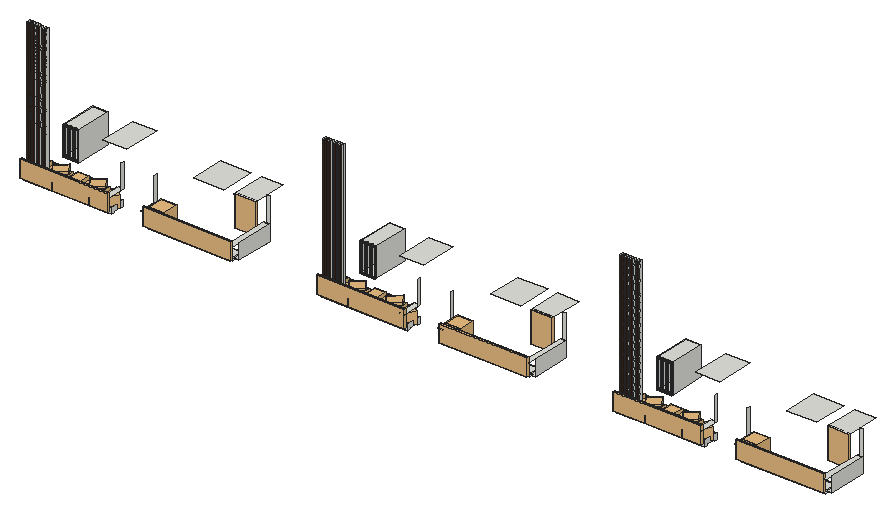
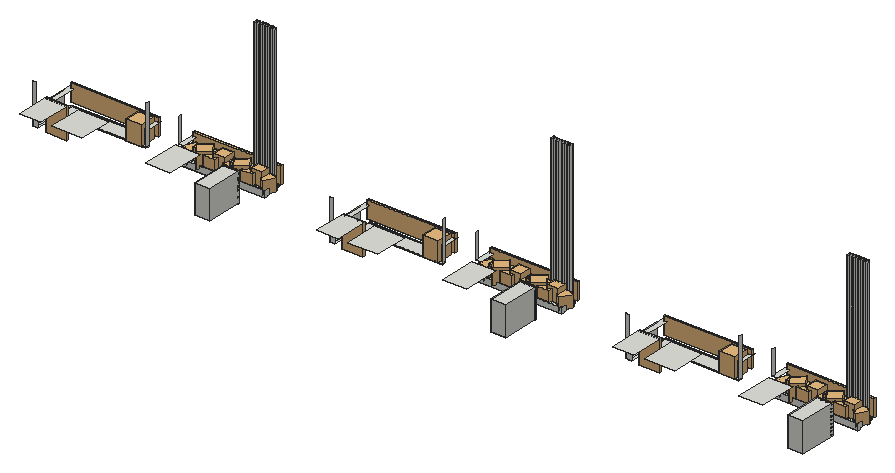
# SketchUp Ruby script. Lengths in inches.
U = 1.inch
M = Sketchup.active_model
def pt(a) = Geom::Point3d.new(a.map { |v| v * U })
def face(e, loops, mat)
  f = e.add_face(loops[0].map { |a| pt(a) })
  loops[1..].each { |l| e.add_face(l.map { |a| pt(a) }).erase! }
  f.material = f.back_material = mat if mat
  f
end
# faces: each face lists its corners as indices into pts; further lists are holes
def faces(e, pts, list, mat = nil) = list.each { |f| face(e, (f[0].is_a?(Array) ? f : [f]).map { |l| l.map { |i| pts[i] } }, mat) }
# xy, xz, yz: faces in a plane at the given z, y or x. An outline is a flat list of corners, or four numbers for a rectangle; further outlines are holes
def ring(l) = l.size == 4 ? [[l[0], l[1]], [l[2], l[1]], [l[2], l[3]], [l[0], l[3]]] : l.each_slice(2).to_a
def flat(e, list, mat, &to3) = list.each { |f| face(e, (f[0].is_a?(Array) ? f : [f]).map { |l| ring(l).map { |u, v| to3.(u, v) } }, mat) }
def xy(e, z, list, mat = nil) = flat(e, list, mat) { |x, y| [x, y, z] }
def xz(e, y, list, mat = nil) = flat(e, list, mat) { |x, z| [x, y, z] }
def yz(e, x, list, mat = nil) = flat(e, list, mat) { |y, z| [x, y, z] }
def lines(e, pts, list) = list.each { |a, b| e.add_line(pt(pts[a]), pt(pts[b])) }
# prism: a flat outline (further loops are holes) pulled along v
def prism(e, loops, v, mat = nil)
  f = face(e, loops, mat); d = Geom::Vector3d.new(v.map { |x| x * U })
  f.pushpull(f.normal.samedirection?(d) ? d.length : -d.length)
end
def box(e, o, s, mat = nil) = prism(e, [[o, [o[0] + s[0], o[1], o[2]], [o[0] + s[0], o[1] + s[1], o[2]], [o[0], o[1] + s[1], o[2]]]], [0, 0, s[2]], mat)
def at(x, y, z, deg = 0) = Geom::Transformation.translation(pt([x, y, z])) * Geom::Transformation.rotation(ORIGIN, Z_AXIS, deg.degrees)
def axes(o, x, y, z) = Geom::Transformation.new([*x, 0, *y, 0, *z, 0, *pt(o).to_a, 1])
def part(name) = M.definitions.add(name)
# library, detail: a bought-in or finely detailed component or shape, given as its bounding box
def library(name, o, s) = part(name).tap { |d| box(d.entities, o, s) }
def detail(e, o, s) = box(e.add_group.entities, o, s)
def put(e, d, t, mat = nil) = e.add_instance(d, t).tap { |i| i.material = mat if mat }
def group(e, t, mat = nil) = e.add_group.tap { |g| g.transformation = t; g.material = mat if mat }.entities
root = M.entities
M.materials.add("Material__1").color = [95, 70, 46]
M.materials.add("Wine2").color = [0, 0, 0]
M.materials["Wine2"].alpha = 0
M.materials.add("[0130_Gainsboro]").color = [39, 45, 50]
M.materials.add("[Wood Floor Parquet]").color = [140, 85, 37]
M.materials.add("[Wood Veneer 01]").color = [51, 28, 15]
c1 = library("Areca palm plant",[0,0,0],[49.1,36.6,54.46])
c2 = library("Group\#74",[-84.69,-90.07,-0.36],[176.51,175.13,171.4])
c3 = library("Group20\#1",[-20.81,-17.08,3.79],[39.86,39.43,37.51])
c4 = library("Group\#130",[-7.34,-1.2,0],[38.67,35.81,49.04])
c5 = library("Group38\#2",[14.01,28.44,-23.43],[18.58,18.32,38.89])
c6 = part("Group\#16")
put(c6.entities,c1,axes([-6.2,158.41,6.08],[0.45017,-0.56191,0],[0.66137,0.52986,0],[0,0,0.72]))
put(c6.entities,c1,axes([-6.2,56.6,6.08],[0.45017,-0.56191,0],[0.66137,0.52986,0],[0,0,0.72]))
put(c6.entities,c2,axes([14.93,145.87,6.05],[-0.04961,-0.08593,0],[0.08593,-0.04961,0],[0,0,0.10522]))
put(c6.entities,c3,axes([18.97,79.98,4.77],[0,0.85,0],[-0.85,0,0],[0,0,0.85]))
put(c6.entities,c2,axes([14.93,173.12,6.05],[-0.04961,-0.08593,0],[0.08593,-0.04961,0],[0,0,0.10522]))
put(c6.entities,c2,axes([14.93,193.18,6.05],[-0.04961,-0.08593,0],[0.08593,-0.04961,0],[0,0,0.10522]))
put(c6.entities,c4,axes([24.9375,89.91,8],[0,0.79,0],[-0.79,0,0],[0,0,0.79]))
put(c6.entities,c5,axes([-4.1,-1.15,28.17],[0.8848,0,0],[0,0.94674,0],[0,0,0.85826]))
g1 = group(c6.entities,at(0,0,0))
xy(g1,0,[[0,0,6,234.8],[30,0,36,234.8]])
xy(g1,3,[[6,0,30,234.8]])
xy(g1,7,[[6,5,30,229.8]],"Material__1")
xy(g1,15,[[[0,0,36,234.8],[6,5,30,229.8]]])
xz(g1,0,[[0,0,6,0,6,3,30,3,30,0,36,0,36,15,0,15]])
xz(g1,5,[[6,7,30,15]])
xz(g1,229.8,[[6,7,30,15]])
xz(g1,234.8,[[0,0,0,15,36,15,36,0,30,0,30,3,6,3,6,0]])
yz(g1,0,[[0,0,234.8,15]])
yz(g1,6,[[0,0,234.8,3],[5,7,229.8,15]])
yz(g1,30,[[0,0,234.8,3],[5,7,229.8,15]])
yz(g1,36,[[0,0,234.8,15]])
put(c6.entities,c2,axes([14.93,91.37,6.05],[-0.04961,-0.08593,0],[0.08593,-0.04961,0],[0,0,0.10522]))
put(c6.entities,c2,axes([14.93,44.05,6.05],[-0.04961,-0.08593,0],[0.08593,-0.04961,0],[0,0,0.10522]))
put(c6.entities,c4,axes([24.9375,191.72,8],[0,0.79,0],[-0.79,0,0],[0,0,0.79]))
put(c6.entities,c5,axes([-4.1,100.66,28.17],[0.8848,0,0],[0,0.94674,0],[0,0,0.85826]))
put(c6.entities,c2,axes([17.19,15.79,6.07],[-0.08133,-0.14087,0],[0.14087,-0.08133,0],[0,0,0.1725]))
put(c6.entities,c2,axes([14.93,71.3,6.05],[-0.04961,-0.08593,0],[0.08593,-0.04961,0],[0,0,0.10522]))
put(c6.entities,c2,axes([17.19,121.23,6.07],[-0.08133,-0.14087,0],[0.14087,-0.08133,0],[0,0,0.1725]))
put(c6.entities,c2,axes([17.19,223.04,6.07],[-0.08133,-0.14087,0],[0.14087,-0.08133,0],[0,0,0.1725]))
put(c6.entities,c3,axes([18.97,181.79,4.77],[0,0.85,0],[-0.85,0,0],[0,0,0.85]))
c7 = library("元件\#5",[-4.39,0,0],[5.37,35.83,90.55])
c8 = library("plant (1)",[-35.72,-28.42,0],[66.31,67.39,84.38])
c9 = library("Glass Railing",[0,0,0],[139.5,4.76,42])
c10 = part("Group\#55")
xy(c10.entities,0,[[0,-0.98,43.07,0],[0,0,43.07,1.4]],"[0130_Gainsboro]")
xy(c10.entities,0.3,[[0.3,-1.43,42.77,-0.98]],"[0130_Gainsboro]")
xy(c10.entities,2.95,[[2.95,-1.43,40.12,-0.63],[2.95,-0.63,40.12,0],[2.95,0,40.12,0.64],[2.95,0.64,40.12,1.4]],"[0130_Gainsboro]")
xy(c10.entities,3.54,[[3.54,-0.63,39.53,0],[3.54,0,39.53,0.64]],"[0130_Gainsboro]")
xy(c10.entities,111.8125,[[3.54,-0.63,39.53,0],[3.54,0,39.53,0.64]],"[0130_Gainsboro]")
xy(c10.entities,112.4,[[2.95,-1.43,40.12,-0.63],[2.95,-0.63,40.12,0],[2.95,0,40.12,0.64],[2.95,0.64,40.12,1.4]],"[0130_Gainsboro]")
xy(c10.entities,115.05,[[0.3,-1.43,42.77,-0.98]],"[0130_Gainsboro]")
xy(c10.entities,115.35,[[0,-0.98,43.07,0],[0,0,43.07,1.4]],"[0130_Gainsboro]")
xz(c10.entities,-1.43,[[[0.3,0.3,42.77,115.05],[2.95,2.95,40.12,112.4]]],"[Wood Veneer 01]")
xz(c10.entities,-0.98,[[[0,0,43.07,115.35],[0.3,0.3,42.77,115.05]]],"[0130_Gainsboro]")
xz(c10.entities,-0.63,[[[2.95,2.95,40.12,112.4],[3.54,3.54,39.53,111.8125]]],"[0130_Gainsboro]")
xz(c10.entities,0,[[3.54,3.54,39.53,111.8125]],"Wine2")
xz(c10.entities,0,[[[0,0,43.07,115.35],[2.95,2.95,40.12,112.4]],[[2.95,2.95,40.12,112.4],[3.54,3.54,39.53,111.8125]]],"[0130_Gainsboro]")
xz(c10.entities,0.64,[[[2.95,2.95,40.12,112.4],[3.54,3.54,39.53,111.8125]]],"[0130_Gainsboro]")
xz(c10.entities,1.4,[[[0,0,43.07,115.35],[2.95,2.95,40.12,112.4]]],"[0130_Gainsboro]")
yz(c10.entities,0,[[-0.98,0,0,115.35],[0,0,1.4,115.35]],"[0130_Gainsboro]")
yz(c10.entities,0.3,[[-1.43,0.3,-0.98,115.05]],"[0130_Gainsboro]")
yz(c10.entities,2.95,[[-1.43,2.95,-0.63,112.4],[-0.63,2.95,0,112.4],[0,2.95,0.64,112.4],[0.64,2.95,1.4,112.4]],"[0130_Gainsboro]")
yz(c10.entities,3.54,[[-0.63,3.54,0,111.8125],[0,3.54,0.64,111.8125]],"[0130_Gainsboro]")
yz(c10.entities,39.53,[[-0.63,3.54,0,111.8125],[0,3.54,0.64,111.8125]],"[0130_Gainsboro]")
yz(c10.entities,40.12,[[-1.43,2.95,-0.63,112.4],[-0.63,2.95,0,112.4],[0,2.95,0.64,112.4],[0.64,2.95,1.4,112.4]],"[0130_Gainsboro]")
yz(c10.entities,42.77,[[-1.43,0.3,-0.98,115.05]],"[0130_Gainsboro]")
yz(c10.entities,43.07,[[-0.98,0,0,115.35],[0,0,1.4,115.35]],"[0130_Gainsboro]")
c11 = part("Component\#21")
put(c11.entities,c10,axes([90.57,1.43,0],[1.05148,0,0],[0,1,0],[0,0,1]))
put(c11.entities,c10,axes([0,1.43,0],[1.05148,0,0],[0,1,0],[0,0,1]))
put(c11.entities,c10,axes([45.29,1.43,0],[1.05148,0,0],[0,1,0],[0,0,1]),"[Wood Veneer 01]")
xy(root,154.75,[[100.18,254.22,106.73,256.84],[106.73,254.22,113.67,256.84],[113.67,254.22,119.31,256.84],[119.31,254.22,126.24,256.84],[126.24,254.22,132.68,256.84],
  [132.68,254.22,139.62,256.84],[139.62,254.22,146.56,256.84],[146.56,254.22,153.49,256.84],[153.49,254.22,303.41,256.84],[409.32,254.22,409.32,255.72,412.47,255.72,412.47,256.84,609.07,256.84,609.07,254.22],
  [833.74,254.22,840.29,256.84],[840.29,254.22,847.23,256.84],[847.23,254.22,852.87,256.84],[852.87,254.22,859.81,256.84],[859.81,254.22,866.24,256.84],
  [866.24,254.22,873.18,256.84],[873.18,254.22,880.12,256.84],[880.12,254.22,887.06,256.84],[887.06,254.22,1036.98,256.84],[1142.89,254.22,1142.89,255.72,1146.03,255.72,1146.03,256.84,1342.64,256.84,1342.64,254.22],
  [1567.3,254.22,1573.86,256.84],[1573.86,254.22,1580.79,256.84],[1580.79,254.22,1586.43,256.84],[1586.43,254.22,1593.37,256.84],[1593.37,254.22,1599.81,256.84],
  [1599.81,254.22,1606.74,256.84],[1606.74,254.22,1613.68,256.84],[1613.68,254.22,1620.62,256.84],[1620.62,254.22,1770.54,256.84],[1876.45,254.22,1876.45,255.72,1879.6,255.72,1879.6,256.84,2076.2,256.84,2076.2,254.22],
  [100.18,256.84,100.18,275.15,303.41,275.15,303.41,256.84,153.49,256.84,153.49,263.78,146.56,263.78,146.56,256.84,139.62,256.84,139.62,263.78,132.68,263.78,132.68,256.84,126.24,256.84,126.24,263.78,119.31,263.78,119.31,256.84,113.67,256.84,113.67,263.78,106.73,263.78,106.73,256.84],[106.73,256.84,113.67,263.78],[119.31,256.84,126.24,263.78],[132.68,256.84,139.62,263.78],[146.56,256.84,153.49,263.78],
  [409.32,256.84,409.32,286.21,396.57,286.21,396.57,293.45,609.07,293.45,609.07,256.84],[609.07,256.84,614.76,266.43],[833.74,256.84,833.74,275.15,1036.98,275.15,1036.98,256.84,887.06,256.84,887.06,263.78,880.12,263.78,880.12,256.84,873.18,256.84,873.18,263.78,866.24,263.78,866.24,256.84,859.81,256.84,859.81,263.78,852.87,263.78,852.87,256.84,847.23,256.84,847.23,263.78,840.29,263.78,840.29,256.84],[840.29,256.84,847.23,263.78],[852.87,256.84,859.81,263.78],
  [866.24,256.84,873.18,263.78],[880.12,256.84,887.06,263.78],[1142.89,256.84,1142.89,286.21,1130.14,286.21,1130.14,293.45,1342.64,293.45,1342.64,256.84],[1342.64,256.84,1348.32,266.43],[1567.3,256.84,1567.3,275.15,1770.54,275.15,1770.54,256.84,1620.62,256.84,1620.62,263.78,1613.68,263.78,1613.68,256.84,1606.74,256.84,1606.74,263.78,1599.81,263.78,1599.81,256.84,1593.37,256.84,1593.37,263.78,1586.43,263.78,1586.43,256.84,1580.79,256.84,1580.79,263.78,1573.86,263.78,1573.86,256.84],
  [1573.86,256.84,1580.79,263.78],[1586.43,256.84,1593.37,263.78],[1599.81,256.84,1606.74,263.78],[1613.68,256.84,1620.62,263.78],[1876.45,256.84,1876.45,286.21,1863.7,286.21,1863.7,293.45,2076.2,293.45,2076.2,256.84],
  [2076.2,256.84,2081.89,266.43],[609.07,266.43,609.07,293.45,614.76,293.45,614.76,361.27,622,361.27,622,266.43],[1342.64,266.43,1342.64,293.45,1348.32,293.45,1348.32,361.27,1355.5625,361.27,1355.5625,266.43],[2076.2,266.43,2076.2,293.45,2081.89,293.45,2081.89,361.27,2089.125,361.27,2089.125,266.43],[609.07,293.45,614.76,361.27],
  [1342.64,293.45,1348.32,361.27],[2076.2,293.45,2081.89,361.27]])
xy(root,154.75,[[409.32,255.72,412.47,256.78],[1142.89,255.72,1146.03,256.78],[1876.45,255.72,1879.6,256.78],[409.32,256.78,412.47,256.84],[1142.89,256.78,1146.03,256.84],
  [1876.45,256.78,1879.6,256.84]],"[Wood Veneer 01]")
xy(root,156.9375,[[409.32,254.22,609.07,256.84],[1142.89,254.22,1342.64,256.84],[1876.45,254.22,2076.2,256.84],[409.32,256.84,609.07,256.84,609.07,293.45,396.57,293.45,396.57,286.21,409.32,286.21],[1142.89,256.84,1342.64,256.84,1342.64,293.45,1130.14,293.45,1130.14,286.21,1142.89,286.21],
  [1876.45,256.84,2076.2,256.84,2076.2,293.45,1863.7,293.45,1863.7,286.21,1876.45,286.21]])
xy(root,158.1875,[[100.18,254.22,106.73,256.84],[113.67,254.22,119.31,256.84],[126.24,254.22,132.68,256.84],[139.62,254.22,146.56,256.84],[153.49,254.22,303.41,256.84],
  [833.74,254.22,840.29,256.84],[847.23,254.22,852.87,256.84],[859.81,254.22,866.24,256.84],[873.18,254.22,880.12,256.84],[887.06,254.22,1036.98,256.84],
  [1567.3,254.22,1573.86,256.84],[1580.79,254.22,1586.43,256.84],[1593.37,254.22,1599.81,256.84],[1606.74,254.22,1613.68,256.84],[1620.62,254.22,1770.54,256.84],
  [100.18,256.84,106.73,256.84,106.73,263.78,113.67,263.78,113.67,256.84,119.31,256.84,119.31,263.78,126.24,263.78,126.24,256.84,132.68,256.84,132.68,263.78,139.62,263.78,139.62,256.84,146.56,256.84,146.56,263.78,153.49,263.78,153.49,256.84,303.41,256.84,303.41,275.15,100.18,275.15],[833.74,256.84,840.29,256.84,840.29,263.78,847.23,263.78,847.23,256.84,852.87,256.84,852.87,263.78,859.81,263.78,859.81,256.84,866.24,256.84,866.24,263.78,873.18,263.78,873.18,256.84,880.12,256.84,880.12,263.78,887.06,263.78,887.06,256.84,1036.98,256.84,1036.98,275.15,833.74,275.15],[1567.3,256.84,1573.86,256.84,1573.86,263.78,1580.79,263.78,1580.79,256.84,1586.43,256.84,1586.43,263.78,1593.37,263.78,1593.37,256.84,1599.81,256.84,1599.81,263.78,1606.74,263.78,1606.74,256.84,1613.68,256.84,1613.68,263.78,1620.62,263.78,1620.62,256.84,1770.54,256.84,1770.54,275.15,1567.3,275.15]])
xy(root,162.74,[[111.92,361.27,149.24,452.58],[845.49,361.27,882.8,452.58],[1579.05,361.27,1616.36,452.58]])
xy(root,193,[[303.35,246.64,315.43,293.45],[396.57,246.64,409.32,286.21],[609.07,246.64,622,361.27],[1036.91,246.64,1049,293.45],[1130.14,246.64,1142.89,286.21],
  [1342.64,246.64,1355.5625,361.27],[1770.48,246.64,1782.56,293.45],[1863.7,246.64,1876.45,286.21],[2076.2,246.64,2089.125,361.27]])
xy(root,230.0625,[[435.49,361.27,509.74,445.08],[1169.05,361.27,1243.3,445.08],[1902.61,361.27,1976.86,445.08]])
xy(root,230.125,[[534.92,361.27,587.67,445.08],[1268.48,361.27,1321.23,445.08],[2002.05,361.27,2054.8,445.08]])
xy(root,234.87,[[111.92,361.27,149.24,452.58],[845.49,361.27,882.8,452.58],[1579.05,361.27,1616.36,452.58]])
xy(root,235.92,[[210.43,361.27,269.1,452.7],[943.99,361.27,1002.66,452.7],[1677.56,361.27,1736.22,452.7]])
xz(root,254.22,[[409.32,154.75,609.07,156.9375],[1142.89,154.75,1342.64,156.9375],[1876.45,154.75,2076.2,156.9375]])
xz(root,254.22,[[100.18,154.75,106.73,158.1875],[106.73,154.75,113.67,506.6875],[113.67,154.75,119.31,158.1875],[119.31,154.75,126.24,506.6875],[126.24,154.75,132.68,158.1875],
  [132.68,154.75,139.62,506.6875],[139.62,154.75,146.56,158.1875],[146.56,154.75,153.49,506.6875],[153.49,154.75,303.41,158.1875],[833.74,154.75,840.29,158.1875],
  [840.29,154.75,847.23,506.6875],[847.23,154.75,852.87,158.1875],[852.87,154.75,859.81,506.6875],[859.81,154.75,866.24,158.1875],[866.24,154.75,873.18,506.6875],
  [873.18,154.75,880.12,158.1875],[880.12,154.75,887.06,506.6875],[887.06,154.75,1036.98,158.1875],[1567.3,154.75,1573.86,158.1875],[1573.86,154.75,1580.79,506.6875],
  [1580.79,154.75,1586.43,158.1875],[1586.43,154.75,1593.37,506.6875],[1593.37,154.75,1599.81,158.1875],[1599.81,154.75,1606.74,506.6875],[1606.74,154.75,1613.68,158.1875],
  [1613.68,154.75,1620.62,506.6875],[1620.62,154.75,1770.54,158.1875]],"[Wood Veneer 01]")
xz(root,256.84,[[100.18,154.75,106.73,158.1875],[106.73,154.75,113.67,506.6875],[113.67,154.75,119.31,158.1875],[119.31,154.75,126.24,506.6875],[126.24,154.75,132.68,158.1875],
  [132.68,154.75,139.62,506.6875],[139.62,154.75,146.56,158.1875],[146.56,154.75,153.49,506.6875],[153.49,154.75,303.41,158.1875],[409.32,154.75,609.07,156.9375],
  [833.74,154.75,840.29,158.1875],[840.29,154.75,847.23,506.6875],[847.23,154.75,852.87,158.1875],[852.87,154.75,859.81,506.6875],[859.81,154.75,866.24,158.1875],
  [866.24,154.75,873.18,506.6875],[873.18,154.75,880.12,158.1875],[880.12,154.75,887.06,506.6875],[887.06,154.75,1036.98,158.1875],[1142.89,154.75,1342.64,156.9375],
  [1567.3,154.75,1573.86,158.1875],[1573.86,154.75,1580.79,506.6875],[1580.79,154.75,1586.43,158.1875],[1586.43,154.75,1593.37,506.6875],[1593.37,154.75,1599.81,158.1875],
  [1599.81,154.75,1606.74,506.6875],[1606.74,154.75,1613.68,158.1875],[1613.68,154.75,1620.62,506.6875],[1620.62,154.75,1770.54,158.1875],[1876.45,154.75,2076.2,156.9375]])
xz(root,263.78,[[106.73,154.75,113.67,158.1875],[119.31,154.75,126.24,158.1875],[132.68,154.75,139.62,158.1875],[146.56,154.75,153.49,158.1875],[840.29,154.75,847.23,158.1875],
  [852.87,154.75,859.81,158.1875],[866.24,154.75,873.18,158.1875],[880.12,154.75,887.06,158.1875],[1573.86,154.75,1580.79,158.1875],[1586.43,154.75,1593.37,158.1875],
  [1599.81,154.75,1606.74,158.1875],[1613.68,154.75,1620.62,158.1875],[106.73,158.1875,113.67,506.6875],[119.31,158.1875,126.24,506.6875],[132.68,158.1875,139.62,506.6875],
  [146.56,158.1875,153.49,506.6875],[840.29,158.1875,847.23,506.6875],[852.87,158.1875,859.81,506.6875],[866.24,158.1875,873.18,506.6875],[880.12,158.1875,887.06,506.6875],
  [1573.86,158.1875,1580.79,506.6875],[1586.43,158.1875,1593.37,506.6875],[1599.81,158.1875,1606.74,506.6875],[1613.68,158.1875,1620.62,506.6875]])
xz(root,275.15,[[100.18,154.75,298.48,158.1875],[298.48,154.75,303.41,158.1875],[833.74,154.75,1032.04,158.1875],[1032.04,154.75,1036.98,158.1875],[1567.3,154.75,1765.6,158.1875],
  [1765.6,154.75,1770.54,158.1875]])
xz(root,286.21,[[396.57,154.75,409.32,156.9375],[1130.14,154.75,1142.89,156.9375],[1863.7,154.75,1876.45,156.9375],[396.57,156.9375,409.32,193],[1130.14,156.9375,1142.89,193],
  [1863.7,156.9375,1876.45,193]])
xz(root,293.45,[[396.57,154.75,609.07,156.9375],[1130.14,154.75,1342.64,156.9375],[1863.7,154.75,2076.2,156.9375]])
xz(root,361.27,[[609.07,154.75,622,193],[1342.64,154.75,1355.5625,193],[2076.2,154.75,2089.125,193],[614.76,193,622,254.6875],[1348.32,193,1355.5625,254.6875],
  [2081.89,193,2089.125,254.6875]])
xz(root,452.58,[[111.92,162.74,149.24,234.87],[845.49,162.74,882.8,234.87],[1579.05,162.74,1616.36,234.87]])
yz(root,100.18,[[254.22,154.75,256.84,158.1875],[256.84,154.75,275.15,158.1875]])
yz(root,106.73,[[254.22,154.75,256.84,158.1875],[256.84,154.75,263.78,158.1875],[254.22,158.1875,256.84,506.6875],[256.84,158.1875,263.78,506.6875]])
yz(root,111.92,[[361.27,162.74,452.58,234.87]])
yz(root,113.67,[[254.22,154.75,256.84,158.1875],[256.84,154.75,263.78,158.1875]])
yz(root,113.67,[[254.22,158.1875,256.84,506.6875],[256.84,158.1875,263.78,506.6875]],"[Wood Veneer 01]")
yz(root,119.31,[[254.22,154.75,256.84,158.1875],[256.84,154.75,263.78,158.1875],[254.22,158.1875,256.84,506.6875],[256.84,158.1875,263.78,506.6875]])
yz(root,126.24,[[254.22,154.75,256.84,158.1875],[256.84,154.75,263.78,158.1875],[254.22,158.1875,256.84,506.6875],[256.84,158.1875,263.78,506.6875]])
yz(root,132.68,[[254.22,154.75,256.84,158.1875],[256.84,154.75,263.78,158.1875],[254.22,158.1875,256.84,506.6875],[256.84,158.1875,263.78,506.6875]])
yz(root,139.62,[[254.22,154.75,256.84,158.1875],[256.84,154.75,263.78,158.1875],[254.22,158.1875,256.84,506.6875],[256.84,158.1875,263.78,506.6875]])
yz(root,146.56,[[254.22,154.75,256.84,158.1875],[256.84,154.75,263.78,158.1875],[254.22,158.1875,256.84,506.6875],[256.84,158.1875,263.78,506.6875]])
yz(root,149.24,[[361.27,162.74,452.58,234.87]])
yz(root,153.49,[[254.22,154.75,256.84,158.1875],[256.84,154.75,263.78,158.1875],[254.22,158.1875,256.84,506.6875],[256.84,158.1875,263.78,506.6875]])
yz(root,303.41,[[254.22,154.75,256.84,158.1875],[256.84,154.75,275.15,158.1875]])
yz(root,315.43,[[286.21,193,293.45,253.5625]])
yz(root,396.57,[[286.21,154.75,293.45,156.9375],[286.21,156.9375,293.45,253.9375]])
yz(root,409.32,[[254.22,154.75,256.84,156.9375],[256.84,154.75,286.21,156.9375]])
yz(root,609.07,[[254.22,154.75,256.84,156.9375],[256.84,154.75,266.43,156.9375],[266.43,154.75,293.45,156.9375]])
yz(root,622,[[266.43,154.75,361.27,193]])
yz(root,833.74,[[254.22,154.75,256.84,158.1875],[256.84,154.75,275.15,158.1875]])
yz(root,840.29,[[254.22,154.75,256.84,158.1875],[256.84,154.75,263.78,158.1875],[254.22,158.1875,256.84,506.6875],[256.84,158.1875,263.78,506.6875]])
yz(root,845.49,[[361.27,162.74,452.58,234.87]])
yz(root,847.23,[[254.22,154.75,256.84,158.1875],[256.84,154.75,263.78,158.1875]])
yz(root,847.23,[[254.22,158.1875,256.84,506.6875],[256.84,158.1875,263.78,506.6875]],"[Wood Veneer 01]")
yz(root,852.87,[[254.22,154.75,256.84,158.1875],[256.84,154.75,263.78,158.1875],[254.22,158.1875,256.84,506.6875],[256.84,158.1875,263.78,506.6875]])
yz(root,859.81,[[254.22,154.75,256.84,158.1875],[256.84,154.75,263.78,158.1875],[254.22,158.1875,256.84,506.6875],[256.84,158.1875,263.78,506.6875]])
yz(root,866.24,[[254.22,154.75,256.84,158.1875],[256.84,154.75,263.78,158.1875],[254.22,158.1875,256.84,506.6875],[256.84,158.1875,263.78,506.6875]])
yz(root,873.18,[[254.22,154.75,256.84,158.1875],[256.84,154.75,263.78,158.1875],[254.22,158.1875,256.84,506.6875],[256.84,158.1875,263.78,506.6875]])
yz(root,880.12,[[254.22,154.75,256.84,158.1875],[256.84,154.75,263.78,158.1875],[254.22,158.1875,256.84,506.6875],[256.84,158.1875,263.78,506.6875]])
yz(root,882.8,[[361.27,162.74,452.58,234.87]])
yz(root,887.06,[[254.22,154.75,256.84,158.1875],[256.84,154.75,263.78,158.1875],[254.22,158.1875,256.84,506.6875],[256.84,158.1875,263.78,506.6875]])
yz(root,1036.98,[[254.22,154.75,256.84,158.1875],[256.84,154.75,275.15,158.1875]])
yz(root,1049,[[286.21,193,293.45,253.5625]])
yz(root,1130.14,[[286.21,154.75,293.45,156.9375],[286.21,156.9375,293.45,253.9375]])
yz(root,1142.89,[[254.22,154.75,256.84,156.9375],[256.84,154.75,286.21,156.9375]])
yz(root,1342.64,[[254.22,154.75,256.84,156.9375],[256.84,154.75,266.43,156.9375],[266.43,154.75,293.45,156.9375]])
yz(root,1355.5625,[[266.43,154.75,361.27,193]])
yz(root,1567.3,[[254.22,154.75,256.84,158.1875],[256.84,154.75,275.15,158.1875]])
yz(root,1573.86,[[254.22,154.75,256.84,158.1875],[256.84,154.75,263.78,158.1875],[254.22,158.1875,256.84,506.6875],[256.84,158.1875,263.78,506.6875]])
yz(root,1579.05,[[361.27,162.74,452.58,234.87]])
yz(root,1580.79,[[254.22,154.75,256.84,158.1875],[256.84,154.75,263.78,158.1875]])
yz(root,1580.79,[[254.22,158.1875,256.84,506.6875],[256.84,158.1875,263.78,506.6875]],"[Wood Veneer 01]")
yz(root,1586.43,[[254.22,154.75,256.84,158.1875],[256.84,154.75,263.78,158.1875],[254.22,158.1875,256.84,506.6875],[256.84,158.1875,263.78,506.6875]])
yz(root,1593.37,[[254.22,154.75,256.84,158.1875],[256.84,154.75,263.78,158.1875],[254.22,158.1875,256.84,506.6875],[256.84,158.1875,263.78,506.6875]])
yz(root,1599.81,[[254.22,154.75,256.84,158.1875],[256.84,154.75,263.78,158.1875],[254.22,158.1875,256.84,506.6875],[256.84,158.1875,263.78,506.6875]])
yz(root,1606.74,[[254.22,154.75,256.84,158.1875],[256.84,154.75,263.78,158.1875],[254.22,158.1875,256.84,506.6875],[256.84,158.1875,263.78,506.6875]])
yz(root,1613.68,[[254.22,154.75,256.84,158.1875],[256.84,154.75,263.78,158.1875],[254.22,158.1875,256.84,506.6875],[256.84,158.1875,263.78,506.6875]])
yz(root,1616.36,[[361.27,162.74,452.58,234.87]])
yz(root,1620.62,[[254.22,154.75,256.84,158.1875],[256.84,154.75,263.78,158.1875],[254.22,158.1875,256.84,506.6875],[256.84,158.1875,263.78,506.6875]])
yz(root,1770.54,[[254.22,154.75,256.84,158.1875],[256.84,154.75,275.15,158.1875]])
yz(root,1782.56,[[286.21,193,293.45,253.5625]])
yz(root,1863.7,[[286.21,154.75,293.45,156.9375],[286.21,156.9375,293.45,253.9375]])
yz(root,1876.45,[[254.22,154.75,256.84,156.9375],[256.84,154.75,286.21,156.9375]])
yz(root,2076.2,[[254.22,154.75,256.84,156.9375],[256.84,154.75,266.43,156.9375],[266.43,154.75,293.45,156.9375]])
yz(root,2089.125,[[266.43,154.75,361.27,193]])
p = [[1032.04,293.45,193],[1032.04,293.46,193],[1765.6,293.45,193],[1765.6,293.46,193],[298.48,293.45,193],[298.48,293.46,193]]
lines(root,p,[[0,1],[2,3],[4,5]])
put(root,c6,axes([1045.33,260.97,150.05],[0,1,0],[-0.9045,0,0],[0,0,1]))
put(root,c6,axes([1778.89,260.97,150.05],[0,1,0],[-0.9045,0,0],[0,0,1]))
put(root,c6,axes([311.76,260.97,150.05],[0,1,0],[-0.9045,0,0],[0,0,1]))
put(root,c7,axes([1269.02,362.12,154.53],[0,-0.89,0],[1.45734,0,0],[0,0,0.83479]),"[Wood Floor Parquet]")
put(root,c7,axes([2002.58,362.12,154.53],[0,-0.89,0],[1.45734,0,0],[0,0,0.83479]),"[Wood Floor Parquet]")
put(root,c7,axes([535.46,362.12,154.53],[0,-0.89,0],[1.45734,0,0],[0,0,0.83479]),"[Wood Floor Parquet]")
put(root,c8,axes([1161.45,271.92,154.75],[0.57,0,0],[0,0.57,0],[0,0,0.57]))
put(root,c8,axes([1895.01,271.92,154.75],[0.57,0,0],[0,0.57,0],[0,0,0.57]))
put(root,c8,axes([427.89,271.92,154.75],[0.57,0,0],[0,0.57,0],[0,0,0.57]))
put(root,c9,axes([829.5,246.93,160.74],[1.55814,0,0],[0,1,0],[0,0,1]))
put(root,c9,axes([1133.0625,246.93,160.74],[1.55814,0,0],[0,1,0],[0,0,1]))
put(root,c9,axes([1866.625,246.93,160.74],[1.55814,0,0],[0,1,0],[0,0,1]))
put(root,c9,axes([1563.0625,246.93,160.74],[1.55814,0,0],[0,1,0],[0,0,1]))
put(root,c9,axes([95.9375,246.93,160.74],[1.55814,0,0],[0,1,0],[0,0,1]))
put(root,c9,axes([399.5,246.93,160.74],[1.55814,0,0],[0,1,0],[0,0,1]))
put(root,c11,axes([845.49,361.27,162.68],[0.27464,0,0],[0,1.2771,0],[0,0,0.62578]))
put(root,c11,axes([1579.05,361.27,162.68],[0.27464,0,0],[0,1.2771,0],[0,0,0.62578]))
put(root,c11,axes([111.92,361.27,162.68],[0.27464,0,0],[0,1.2771,0],[0,0,0.62578]))
